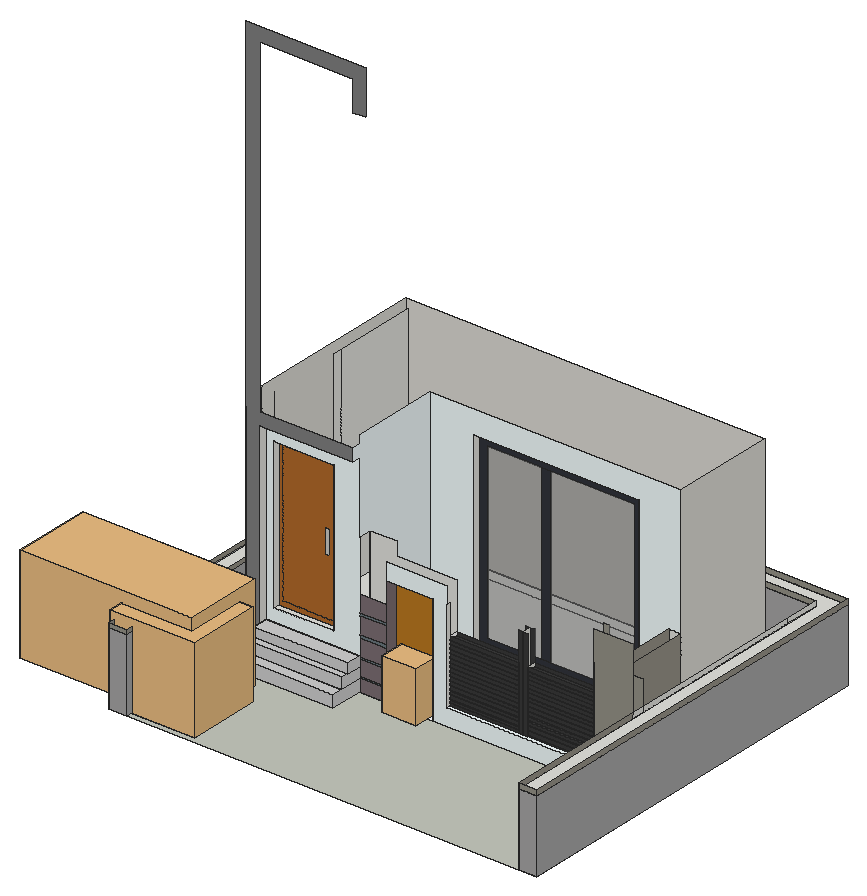
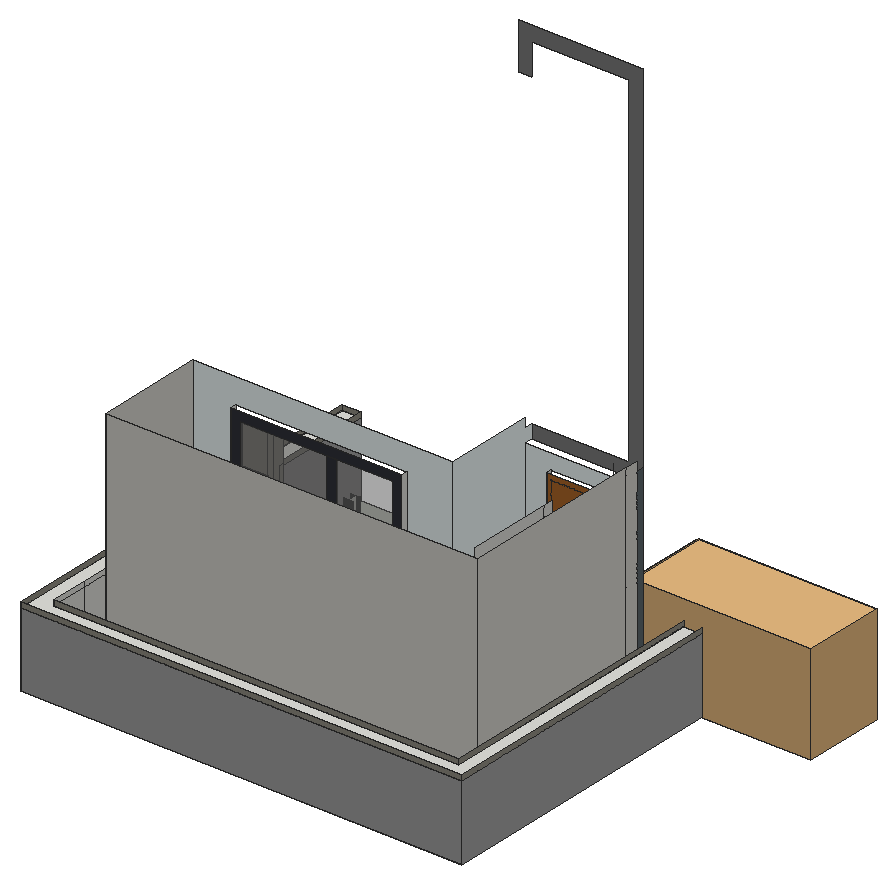
# SketchUp Ruby script. Lengths in inches.
U = 1.inch
M = Sketchup.active_model
def pt(a) = Geom::Point3d.new(a.map { |v| v * U })
def face(e, loops, mat)
  f = e.add_face(loops[0].map { |a| pt(a) })
  loops[1..].each { |l| e.add_face(l.map { |a| pt(a) }).erase! }
  f.material = f.back_material = mat if mat
  f
end
# faces: each face lists its corners as indices into pts; further lists are holes
def faces(e, pts, list, mat = nil) = list.each { |f| face(e, (f[0].is_a?(Array) ? f : [f]).map { |l| l.map { |i| pts[i] } }, mat) }
# xy, xz, yz: faces in a plane at the given z, y or x. An outline is a flat list of corners, or four numbers for a rectangle; further outlines are holes
def ring(l) = l.size == 4 ? [[l[0], l[1]], [l[2], l[1]], [l[2], l[3]], [l[0], l[3]]] : l.each_slice(2).to_a
def flat(e, list, mat, &to3) = list.each { |f| face(e, (f[0].is_a?(Array) ? f : [f]).map { |l| ring(l).map { |u, v| to3.(u, v) } }, mat) }
def xy(e, z, list, mat = nil) = flat(e, list, mat) { |x, y| [x, y, z] }
def xz(e, y, list, mat = nil) = flat(e, list, mat) { |x, z| [x, y, z] }
def yz(e, x, list, mat = nil) = flat(e, list, mat) { |y, z| [x, y, z] }
def lines(e, pts, list) = list.each { |a, b| e.add_line(pt(pts[a]), pt(pts[b])) }
# prism: a flat outline (further loops are holes) pulled along v
def prism(e, loops, v, mat = nil)
  f = face(e, loops, mat); d = Geom::Vector3d.new(v.map { |x| x * U })
  f.pushpull(f.normal.samedirection?(d) ? d.length : -d.length)
end
def box(e, o, s, mat = nil) = prism(e, [[o, [o[0] + s[0], o[1], o[2]], [o[0] + s[0], o[1] + s[1], o[2]], [o[0], o[1] + s[1], o[2]]]], [0, 0, s[2]], mat)
def at(x, y, z, deg = 0) = Geom::Transformation.translation(pt([x, y, z])) * Geom::Transformation.rotation(ORIGIN, Z_AXIS, deg.degrees)
def axes(o, x, y, z) = Geom::Transformation.new([*x, 0, *y, 0, *z, 0, *pt(o).to_a, 1])
def part(name) = M.definitions.add(name)
# library, detail: a bought-in or finely detailed component or shape, given as its bounding box
def library(name, o, s) = part(name).tap { |d| box(d.entities, o, s) }
def detail(e, o, s) = box(e.add_group.entities, o, s)
def put(e, d, t, mat = nil) = e.add_instance(d, t).tap { |i| i.material = mat if mat }
def group(e, t, mat = nil) = e.add_group.tap { |g| g.transformation = t; g.material = mat if mat }.entities
root = M.entities
M.materials.add("[0133_Gray]").color = [128, 128, 128]
M.materials.add("[Asphalt New]").color = [124, 111, 115]
M.materials.add("[Blinds Weave]").color = [186, 120, 33]
M.materials.add("[Carrera Marble]").color = [207, 207, 207]
M.materials.add("[Color M00]").color = [255, 255, 255]
M.materials.add("[Color M07]").color = [58, 58, 58]
M.materials.add("[Formica Graystone]").color = [149, 146, 135]
M.materials.add("[Formica Laminate Dark]").color = [50, 53, 60]
M.materials.add("[Formica Speckled Grey]").color = [107, 120, 127]
M.materials.add("[Formica Speckled Grey]1").color = [94, 105, 111]
M.materials.add("[Pavers with Grass Herringbone]").color = [197, 201, 190]
M.materials.add("[Stone Vein Gray]").color = [166, 165, 165]
M.materials.add("[Terrazzo Tile Light]").color = [219, 217, 210]
M.materials.add("[Translucent Glass Gray]").color = [128, 128, 128]
M.materials["[Translucent Glass Gray]"].alpha = 0.5
M.materials.add("[White Subway Tile]").color = [243, 252, 253]
M.materials.add("[Wood Bamboo]").color = [177, 105, 43]
c1 = library("SPIKED_SUCCULENT_skp2020",[-8.43,-6.07,-0.04],[14.15,14.04,18.09])
c2 = library("Flora+17",[-57.52,158.6,-38.64],[66.99,62.88,77.28])
c3 = library("Sem+nome",[-20.92,-6.25,0],[92.79,42.83,52.11])
xy(root,0,[[0,0,0,210.34,230.95,210.34,230.95,0,221.32,0,221.32,200.71,9.63,200.71,9.63,0],[22.92,59.54,73.48,77.29],[15.28,77.29,15.28,181.19,221.32,181.19,221.32,77.29,113.16,77.29,113.16,83.29,88.1,83.29,88.1,77.29]])
xy(root,0,[[88.1,77.29,113.16,83.29]],"[Color M00]")
xy(root,0,[[[9.63,0,221.32,200.71],[22.92,59.54,73.48,59.54,73.48,77.29,15.28,77.29,15.28,72.92,22.92,72.92],[88.1,77.29,113.16,83.29]]],"[Pavers with Grass Herringbone]")
xy(root,6.48,[[22.92,65.48,73.48,77.29]])
xy(root,6.48,[[22.92,59.54,73.48,65.48]],"[Carrera Marble]")
xy(root,9,[[120.8,79.26,158.09,83.94],[158.09,79.26,160.4375,83.94],[160.4375,79.26,162.78,83.94],[15.28,83.94,15.28,181.19,209.59,181.19,209.59,124.55,202.93,124.55,202.93,174.54,21.94,174.54,21.94,83.94],[73.48,83.94,202.93,83.94,202.93,124.55,186.72,124.55,186.72,127.86,97.58,127.86,97.58,124.55,73.48,124.55],
  [202.93,83.94,209.59,124.55],[209.59,83.94,221.32,124.55],[21.94,124.55,21.94,129.24,202.93,129.24,202.93,124.55,186.72,124.55,186.72,127.86,97.58,127.86,97.58,124.55],[209.59,124.55,221.32,181.19],[21.94,129.24,202.93,174.54]])
xy(root,9,[[162.78,79.26,200.125,83.94]],"[Color M07]")
xy(root,9,[[120.8,77.29,200.125,79.26]],"[White Subway Tile]")
xy(root,9.77,[[162.78,79.26,200.125,83.94]])
xy(root,10.46,[[120.8,79.26,158.09,83.94]],"[Color M07]")
xy(root,10.73,[[120.8,79.26,158.09,83.94]],"[Color M00]")
xy(root,11.53,[[162.78,79.26,200.125,83.94]],"[Color M07]")
xy(root,12.15,[[162.78,79.26,200.125,83.94]])
xy(root,12.22,[[120.8,79.26,158.09,83.94]],"[Color M07]")
xy(root,12.39,[[22.92,69.29,73.48,77.29]])
xy(root,12.39,[[22.92,65.48,73.48,69.29]],"[Carrera Marble]")
xy(root,12.65,[[120.8,79.26,158.09,83.94]],"[Color M00]")
xy(root,13.91,[[162.78,79.26,200.125,83.94]],"[Color M07]")
xy(root,14.41,[[120.8,79.26,158.09,83.94]],"[Color M07]")
xy(root,14.52,[[162.78,79.26,200.125,83.94]],"[Color M07]")
xy(root,14.84,[[120.8,79.26,158.09,83.94]],"[Color M07]")
xy(root,16.28,[[162.78,79.26,200.125,83.94]],"[Color M07]")
xy(root,16.59,[[120.8,79.26,158.09,83.94]],"[Color M07]")
xy(root,16.9,[[162.78,79.26,200.125,83.94]],"[Color M07]")
xy(root,17.02,[[120.8,79.26,158.09,83.94]],"[Color M07]")
xy(root,17.57,[[22.92,69.29,73.48,77.29]],"[Carrera Marble]")
xy(root,18.66,[[162.78,79.26,200.125,83.94]],"[Color M07]")
xy(root,18.78,[[120.8,79.26,158.09,83.94]],"[Color M07]")
xy(root,19.21,[[120.8,79.26,158.09,83.94]],"[Color M07]")
xy(root,19.27,[[162.78,79.26,200.125,83.94]],"[Color M07]")
xy(root,20.97,[[120.8,79.26,158.09,83.94]],"[Color M07]")
xy(root,21.03,[[162.78,79.26,200.125,83.94]],"[Color M07]")
xy(root,21.4,[[120.8,79.26,158.09,83.94]],"[Color M07]")
xy(root,21.65,[[162.78,79.26,200.125,83.94]],"[Color M07]")
xy(root,23.16,[[120.8,79.26,158.09,83.94]],"[Color M07]")
xy(root,23.41,[[162.78,79.26,200.125,83.94]],"[Color M07]")
xy(root,23.59,[[120.8,79.26,158.09,83.94]],"[Color M07]")
xy(root,24.02,[[162.78,79.26,200.125,83.94]],"[Color M07]")
xy(root,24.78,[[27.2,77.29,59.83,80.42]])
xy(root,25.34,[[120.8,79.26,158.09,83.94]],"[Color M07]")
xy(root,25.77,[[120.8,79.26,158.09,83.94]],"[Color M07]")
xy(root,25.78,[[162.78,79.26,200.125,83.94]],"[Color M07]")
xy(root,26.15,[[162.78,79.26,200.125,83.94]],"[Color M07]")
xy(root,27.53,[[120.8,79.26,158.09,83.94]],"[Color M07]")
xy(root,27.91,[[162.78,79.26,200.125,83.94]],"[Color M07]")
xy(root,27.96,[[120.8,79.26,158.09,83.94]],"[Color M07]")
xy(root,28.27,[[162.78,79.26,200.125,83.94]],"[Color M07]")
xy(root,29.72,[[120.8,79.26,158.09,83.94]],"[Color M07]")
xy(root,30.03,[[162.78,79.26,200.125,83.94]],"[Color M07]")
xy(root,30.15,[[120.8,79.26,158.09,83.94]],"[Color M07]")
xy(root,30.4,[[162.78,79.26,200.125,83.94]],"[Color M07]")
xy(root,31.91,[[120.8,79.26,158.09,83.94]],"[Color M07]")
xy(root,32.16,[[162.78,79.26,200.125,83.94]],"[Color M07]")
xy(root,32.34,[[120.8,79.26,158.09,83.94]],"[Color M07]")
xy(root,32.52,[[162.78,79.26,200.125,83.94]],"[Color M07]")
xy(root,34.09,[[120.8,79.26,158.09,83.94]],"[Color M07]")
xy(root,34.28,[[162.78,79.26,200.125,83.94]],"[Color M07]")
xy(root,34.52,[[120.8,79.26,158.09,83.94]],"[Color M07]")
xy(root,34.65,[[162.78,79.26,200.125,83.94]],"[Color M07]")
xy(root,36.28,[[120.8,79.26,158.09,83.94]],"[Color M07]")
xy(root,36.41,[[162.78,79.26,200.125,83.94]],"[Color M07]")
xy(root,36.71,[[120.8,79.26,158.09,83.94],[162.78,79.26,200.125,83.94]],"[Color M07]")
xy(root,38.47,[[120.8,79.26,158.09,83.94],[162.78,79.26,200.125,83.94]],"[Color M07]")
xy(root,38.77,[[162.78,79.26,200.125,83.94]],"[Color M07]")
xy(root,38.9,[[120.8,79.26,158.09,83.94]],"[Color M07]")
xy(root,39.1875,[[0,0,0,210.34,230.95,210.34,230.95,0,221.32,0,221.32,200.71,9.63,200.71,9.63,0]])
xy(root,40.53,[[162.78,79.26,200.125,83.94]],"[Color M07]")
xy(root,40.66,[[120.8,79.26,158.09,83.94]],"[Color M07]")
xy(root,40.84,[[200.125,79.26,200.1875,83.94]])
xy(root,40.84,[[162.78,79.26,200.125,83.94]],"[Color M07]")
xy(root,41.09,[[120.8,79.26,158.09,83.94]],"[Color M07]")
xz(root,0,[[0,39.1875,9.63,41.8125],[221.32,39.1875,230.95,41.8125]],"[Formica Graystone]")
xz(root,0,[[0,0,9.63,39.1875],[221.32,0,230.95,39.1875]],"[Stone Vein Gray]")
xz(root,59.54,[[22.92,0,73.48,6.48]],"[Carrera Marble]")
xz(root,65.48,[[22.92,6.48,73.48,12.39]],"[Carrera Marble]")
xz(root,69.29,[[22.92,12.39,73.48,17.57]],"[Carrera Marble]")
xz(root,72.92,[[15.28,0,22.92,0,22.92,113.3,73.48,113.3,73.48,120,22.92,120,22.92,298.85,73.48,298.85,73.48,282.625,80.125,282.625,80.125,306.8125,15.28,306.8125]],"[0133_Gray]")
xz(root,77.29,[[15.28,0,15.28,120,20.35,120,20.35,113.3,22.92,113.3,22.92,0],[22.92,0,73.48,6.48],[22.92,6.48,73.48,12.39],[22.92,12.39,73.48,17.57]])
xz(root,77.29,[[73.48,0,88.1,6.88],[73.48,7.76,88.1,16],[73.48,17.13,88.1,26.25],[73.48,27.94,88.1,37.0625],[73.48,38.44,88.1,47.5625]],"[Asphalt New]")
xz(root,77.29,[[200.125,0,221.32,75.3125]],"[Formica Graystone]")
xz(root,77.29,[[73.48,6.88,88.1,7.76],[73.48,16,88.1,17.13],[73.48,26.25,88.1,27.94],[73.48,37.0625,88.1,38.44]],"[Formica Speckled Grey]")
xz(root,77.29,[[113.16,0,200.125,0,200.125,9,120.8,9,120.8,68,88.1,68,88.1,58.88,113.16,58.88],[[22.92,17.57,73.48,113.3],[27.2,24.78,59.83,105.34]]],"[White Subway Tile]")
xz(root,79.26,[[200.125,40.84,200.1875,42.59]])
xz(root,79.26,[[120.8,9,158.09,10.46],[158.09,9,160.4375,58.88],[160.4375,9,162.78,58.88],[162.78,9.77,200.125,11.53],[120.8,10.73,158.09,12.22],
  [162.78,12.15,200.125,13.91],[120.8,12.65,158.09,14.41],[162.78,14.52,200.125,16.28],[120.8,14.84,158.09,16.59],[162.78,16.9,200.125,18.66],
  [120.8,17.02,158.09,18.78],[120.8,19.21,158.09,20.97],[162.78,19.27,200.125,21.03],[120.8,21.4,158.09,23.16],[162.78,21.65,200.125,23.41],
  [120.8,23.59,158.09,25.34],[162.78,24.02,200.125,25.78],[120.8,25.77,158.09,27.53],[162.78,26.15,200.125,27.91],[120.8,27.96,158.09,29.72],
  [162.78,28.27,200.125,30.03],[120.8,30.15,158.09,31.91],[162.78,30.4,200.125,32.16],[120.8,32.34,158.09,34.09],[162.78,32.52,200.125,34.28],
  [120.8,34.52,158.09,36.28],[162.78,34.65,200.125,36.41],[120.8,36.71,158.09,38.47],[162.78,36.71,200.125,38.47],[162.78,38.77,200.125,40.53],
  [120.8,38.9,158.09,40.66],[162.78,40.84,200.125,42.59],[120.8,41.09,158.09,42.84]],"[Color M07]")
xz(root,80.42,[[[27.2,24.78,59.83,105.34],[29.59,27.16,57.44,102.95]],[[29.59,27.16,57.44,102.95],[52.45,57.88,54.7,71.19]]],"[Wood Bamboo]")
xz(root,83.29,[[88.1,0,113.16,58.88]],"[Blinds Weave]")
xz(root,83.94,[[73.48,9,73.48,75.3125,88.1,75.3125,88.1,68,120.8,68,120.8,9],[202.93,9,209.59,55.3125],[200.125,40.84,200.1875,42.59]])
xz(root,83.94,[[120.8,9,158.09,10.46],[158.09,9,160.4375,58.88],[160.4375,9,162.78,58.88],[162.78,9.77,200.125,11.53],[120.8,10.73,158.09,12.22],
  [162.78,12.15,200.125,13.91],[120.8,12.65,158.09,14.41],[162.78,14.52,200.125,16.28],[120.8,14.84,158.09,16.59],[162.78,16.9,200.125,18.66],
  [120.8,17.02,158.09,18.78],[120.8,19.21,158.09,20.97],[162.78,19.27,200.125,21.03],[120.8,21.4,158.09,23.16],[162.78,21.65,200.125,23.41],
  [120.8,23.59,158.09,25.34],[162.78,24.02,200.125,25.78],[120.8,25.77,158.09,27.53],[162.78,26.15,200.125,27.91],[120.8,27.96,158.09,29.72],
  [162.78,28.27,200.125,30.03],[120.8,30.15,158.09,31.91],[162.78,30.4,200.125,32.16],[120.8,32.34,158.09,34.09],[162.78,32.52,200.125,34.28],
  [120.8,34.52,158.09,36.28],[162.78,34.65,200.125,36.41],[120.8,36.71,158.09,38.47],[162.78,36.71,200.125,38.47],[162.78,38.77,200.125,40.53],
  [120.8,38.9,158.09,40.66],[162.78,40.84,200.125,42.59],[120.8,41.09,158.09,42.84]],"[Color M07]")
xz(root,83.94,[[200.125,9,200.125,40.84,200.1875,40.84,200.1875,42.59,200.125,42.59,200.125,75.3125,202.93,75.3125,202.93,9],[209.59,9,221.32,55.3125]],"[Formica Graystone]")
xz(root,124.55,[[202.93,9,209.59,55.3125]])
xz(root,124.55,[[73.48,9,97.58,9,97.58,112.0625,186.72,112.0625,186.72,9,202.93,9,202.93,55.3125,209.59,55.3125,209.59,124.8125,73.48,124.8125]],"[White Subway Tile]")
xz(root,127.86,[[[97.58,9,186.72,112.0625],[102.43,13.86,181.86,107.2]],[131.34,13.86,136.54,107.2]],"[Formica Laminate Dark]")
xz(root,127.86,[[102.43,13.86,131.34,107.2],[136.54,13.86,181.86,107.2]],"[Translucent Glass Gray]")
xz(root,181.19,[[15.28,0,221.32,9]])
xz(root,181.19,[[15.28,9,209.59,124.8125]],"[Terrazzo Tile Light]")
xz(root,200.71,[[9.63,39.1875,221.32,41.8125]],"[Formica Graystone]")
xz(root,200.71,[[9.63,0,221.32,39.1875]],"[Stone Vein Gray]")
xz(root,210.34,[[0,39.1875,230.95,41.8125]],"[Formica Graystone]")
xz(root,210.34,[[0,0,230.95,39.1875]],"[Stone Vein Gray]")
yz(root,0,[[0,39.1875,210.34,41.8125]],"[Formica Graystone]")
yz(root,0,[[0,0,210.34,39.1875]],"[Stone Vein Gray]")
yz(root,9.63,[[0,39.1875,200.71,41.8125]],"[Formica Graystone]")
yz(root,9.63,[[0,0,200.71,39.1875]],"[Stone Vein Gray]")
yz(root,15.28,[[77.29,0,181.19,9]])
yz(root,15.28,[[72.92,0,77.29,120]],"[Formica Speckled Grey]1")
yz(root,15.28,[[77.29,9,83.94,124.8125],[83.94,9,181.19,124.8125]],"[Terrazzo Tile Light]")
yz(root,21.94,[[124.55,9,129.24,124.8125],[129.24,9,174.54,124.8125]])
yz(root,22.92,[[72.92,0,77.29,6.48],[72.92,6.48,77.29,12.39],[72.92,12.39,77.29,17.57],[72.92,17.57,77.29,113.3]])
yz(root,22.92,[[59.54,0,72.92,6.48],[65.48,6.48,72.92,12.39],[69.29,12.39,72.92,17.57]],"[Carrera Marble]")
yz(root,27.2,[[77.29,24.78,80.42,105.34]])
yz(root,59.83,[[77.29,24.78,80.42,105.34]])
yz(root,73.48,[[59.54,0,77.29,6.48],[65.48,6.48,77.29,12.39],[69.29,12.39,77.29,17.57]],"[Carrera Marble]")
yz(root,73.48,[[83.94,9,124.55,9,124.55,124.8125,77.29,124.8125,77.29,120,72.92,120,72.92,113.3,77.29,113.3,77.29,75.3125,83.94,75.3125]],"[White Subway Tile]")
yz(root,88.1,[[77.29,0,83.29,58.88]],"[Asphalt New]")
yz(root,97.58,[[124.55,9,127.86,112.0625]])
yz(root,113.16,[[77.29,0,83.29,58.88]])
yz(root,120.8,[[77.29,9,79.26,58.88],[79.26,9,83.94,10.46],[79.26,12.22,83.94,12.65],[79.26,14.41,83.94,14.84],[79.26,16.59,83.94,17.02],
  [79.26,18.78,83.94,19.21],[79.26,20.97,83.94,21.4],[79.26,23.16,83.94,23.59],[79.26,25.34,83.94,25.77],[79.26,27.53,83.94,27.96],
  [79.26,29.72,83.94,30.15],[79.26,31.91,83.94,32.34],[79.26,34.09,83.94,34.52],[79.26,36.28,83.94,36.71],[79.26,38.47,83.94,38.9],
  [79.26,40.66,83.94,41.09]])
yz(root,120.8,[[79.26,10.46,83.94,10.73],[79.26,10.73,83.94,12.22],[79.26,12.65,83.94,14.41],[79.26,14.84,83.94,16.59],[79.26,17.02,83.94,18.78],
  [79.26,19.21,83.94,20.97],[79.26,21.4,83.94,23.16],[79.26,23.59,83.94,25.34],[79.26,25.77,83.94,27.53],[79.26,27.96,83.94,29.72],
  [79.26,30.15,83.94,31.91],[79.26,32.34,83.94,34.09],[79.26,34.52,83.94,36.28],[79.26,36.71,83.94,38.47],[79.26,38.9,83.94,40.66],
  [79.26,41.09,83.94,42.84]],"[Color M00]")
yz(root,158.09,[[79.26,10.46,83.94,10.73],[79.26,12.22,83.94,12.65],[79.26,14.41,83.94,14.84],[79.26,16.59,83.94,17.02],[79.26,18.78,83.94,19.21],
  [79.26,20.97,83.94,21.4],[79.26,23.16,83.94,23.59],[79.26,25.34,83.94,25.77],[79.26,27.53,83.94,27.96],[79.26,29.72,83.94,30.15],
  [79.26,31.91,83.94,32.34],[79.26,34.09,83.94,34.52],[79.26,36.28,83.94,36.71],[79.26,38.47,83.94,38.9],[79.26,40.66,83.94,41.09]])
yz(root,158.09,[[79.26,10.73,83.94,12.22],[79.26,12.65,83.94,14.41],[79.26,14.84,83.94,16.59],[79.26,17.02,83.94,18.78],[79.26,19.21,83.94,20.97],
  [79.26,21.4,83.94,23.16],[79.26,23.59,83.94,25.34],[79.26,25.77,83.94,27.53],[79.26,27.96,83.94,29.72],[79.26,30.15,83.94,31.91],
  [79.26,32.34,83.94,34.09],[79.26,34.52,83.94,36.28],[79.26,36.71,83.94,38.47],[79.26,38.9,83.94,40.66],[79.26,41.09,83.94,42.84]],"[Color M00]")
yz(root,160.4375,[[79.26,9,83.94,58.88]])
yz(root,162.78,[[79.26,9,83.94,9.77],[79.26,9.77,83.94,11.53],[79.26,11.53,83.94,12.15],[79.26,12.15,83.94,13.91],[79.26,13.91,83.94,14.52],
  [79.26,14.52,83.94,16.28],[79.26,16.28,83.94,16.9],[79.26,16.9,83.94,18.66],[79.26,18.66,83.94,19.27],[79.26,19.27,83.94,21.03],
  [79.26,21.03,83.94,21.65],[79.26,21.65,83.94,23.41],[79.26,23.41,83.94,24.02],[79.26,24.02,83.94,25.78],[79.26,25.78,83.94,26.15],
  [79.26,26.15,83.94,27.91],[79.26,27.91,83.94,28.27],[79.26,28.27,83.94,30.03],[79.26,30.03,83.94,30.4],[79.26,30.4,83.94,32.16],
  [79.26,32.16,83.94,32.52],[79.26,32.52,83.94,34.28],[79.26,34.28,83.94,34.65],[79.26,34.65,83.94,36.41],[79.26,36.41,83.94,36.71],
  [79.26,36.71,83.94,38.47],[79.26,38.47,83.94,38.77],[79.26,38.77,83.94,40.53],[79.26,40.53,83.94,40.84],[79.26,40.84,83.94,42.59]])
yz(root,186.72,[[124.55,9,127.86,112.0625]])
yz(root,200.125,[[79.26,9,83.94,9.77],[79.26,9.77,83.94,11.53],[79.26,11.53,83.94,12.15],[79.26,12.15,83.94,13.91],[79.26,13.91,83.94,14.52],
  [79.26,14.52,83.94,16.28],[79.26,16.28,83.94,16.9],[79.26,16.9,83.94,18.66],[79.26,18.66,83.94,19.27],[79.26,19.27,83.94,21.03],
  [79.26,21.03,83.94,21.65],[79.26,21.65,83.94,23.41],[79.26,23.41,83.94,24.02],[79.26,24.02,83.94,25.78],[79.26,25.78,83.94,26.15],
  [79.26,26.15,83.94,27.91],[79.26,27.91,83.94,28.27],[79.26,28.27,83.94,30.03],[79.26,30.03,83.94,30.4],[79.26,30.4,83.94,32.16],
  [79.26,32.16,83.94,32.52],[79.26,32.52,83.94,34.28],[79.26,34.28,83.94,34.65],[79.26,34.65,83.94,36.41],[79.26,36.41,83.94,36.71],
  [79.26,36.71,83.94,38.47],[79.26,38.47,83.94,38.77],[79.26,38.77,83.94,40.53],[79.26,40.53,83.94,40.84],[79.26,40.84,83.94,42.59]])
yz(root,200.125,[[77.29,9,79.26,58.88]],"[Formica Graystone]")
yz(root,200.1875,[[79.26,40.84,83.94,42.59]])
yz(root,202.93,[[83.94,9,124.55,55.3125]],"[Formica Graystone]")
yz(root,209.59,[[83.94,9,124.55,55.3125]],"[Formica Graystone]")
yz(root,209.59,[[124.55,9,181.19,124.8125]],"[Terrazzo Tile Light]")
yz(root,221.32,[[77.29,0,181.19,9],[181.19,0,200.71,39.1875],[77.29,9,83.94,39.1875],[83.94,9,181.19,39.1875],[77.29,39.1875,83.94,41.8125],
  [83.94,39.1875,181.19,41.8125],[181.19,39.1875,200.71,41.8125]])
yz(root,221.32,[[0,39.1875,77.29,41.8125]],"[Formica Graystone]")
yz(root,221.32,[[0,0,77.29,39.1875]],"[Stone Vein Gray]")
yz(root,230.95,[[0,39.1875,210.34,41.8125]],"[Formica Graystone]")
yz(root,230.95,[[0,0,210.34,39.1875]],"[Stone Vein Gray]")
p = [[21.94,83.94,9],[21.94,83.94,124.8125]]
lines(root,p,[[0,1]])
put(root,c1,axes([102.43,75.76,0.0625],[1.3,0,0],[0,1,0],[0,0,1.5]))
put(root,c2,axes([37.04,-96.73,22.91],[0.68,0,0],[0,0.63,0],[0,0,0.5928]))
put(root,c3,at(-35.99,17.01,0))
